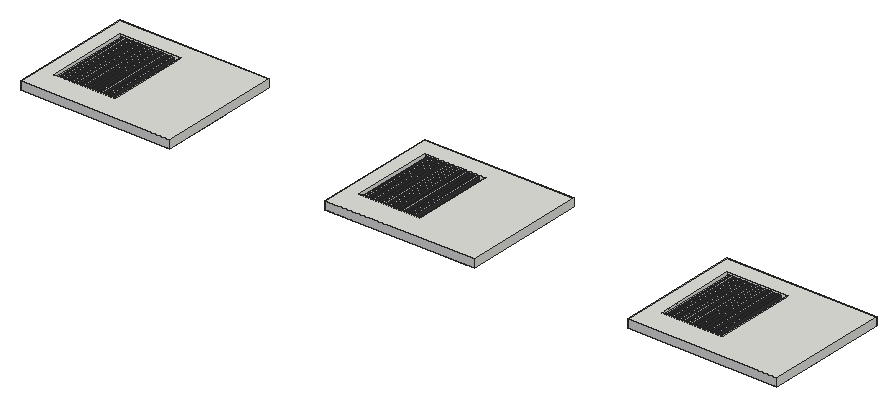
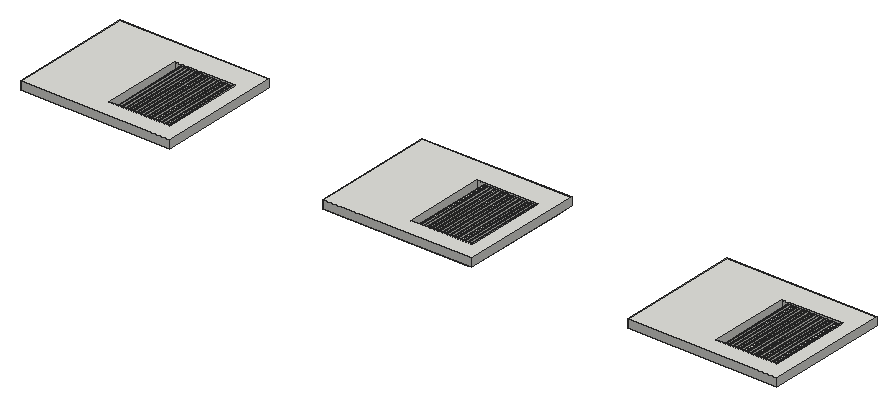
# SketchUp Ruby script. Lengths in inches.
U = 1.inch
M = Sketchup.active_model
def pt(a) = Geom::Point3d.new(a.map { |v| v * U })
def face(e, loops, mat)
  f = e.add_face(loops[0].map { |a| pt(a) })
  loops[1..].each { |l| e.add_face(l.map { |a| pt(a) }).erase! }
  f.material = f.back_material = mat if mat
  f
end
# faces: each face lists its corners as indices into pts; further lists are holes
def faces(e, pts, list, mat = nil) = list.each { |f| face(e, (f[0].is_a?(Array) ? f : [f]).map { |l| l.map { |i| pts[i] } }, mat) }
# xy, xz, yz: faces in a plane at the given z, y or x. An outline is a flat list of corners, or four numbers for a rectangle; further outlines are holes
def ring(l) = l.size == 4 ? [[l[0], l[1]], [l[2], l[1]], [l[2], l[3]], [l[0], l[3]]] : l.each_slice(2).to_a
def flat(e, list, mat, &to3) = list.each { |f| face(e, (f[0].is_a?(Array) ? f : [f]).map { |l| ring(l).map { |u, v| to3.(u, v) } }, mat) }
def xy(e, z, list, mat = nil) = flat(e, list, mat) { |x, y| [x, y, z] }
def xz(e, y, list, mat = nil) = flat(e, list, mat) { |x, z| [x, y, z] }
def yz(e, x, list, mat = nil) = flat(e, list, mat) { |y, z| [x, y, z] }
def lines(e, pts, list) = list.each { |a, b| e.add_line(pt(pts[a]), pt(pts[b])) }
# prism: a flat outline (further loops are holes) pulled along v
def prism(e, loops, v, mat = nil)
  f = face(e, loops, mat); d = Geom::Vector3d.new(v.map { |x| x * U })
  f.pushpull(f.normal.samedirection?(d) ? d.length : -d.length)
end
def box(e, o, s, mat = nil) = prism(e, [[o, [o[0] + s[0], o[1], o[2]], [o[0] + s[0], o[1] + s[1], o[2]], [o[0], o[1] + s[1], o[2]]]], [0, 0, s[2]], mat)
def at(x, y, z, deg = 0) = Geom::Transformation.translation(pt([x, y, z])) * Geom::Transformation.rotation(ORIGIN, Z_AXIS, deg.degrees)
def axes(o, x, y, z) = Geom::Transformation.new([*x, 0, *y, 0, *z, 0, *pt(o).to_a, 1])
def part(name) = M.definitions.add(name)
# library, detail: a bought-in or finely detailed component or shape, given as its bounding box
def library(name, o, s) = part(name).tap { |d| box(d.entities, o, s) }
def detail(e, o, s) = box(e.add_group.entities, o, s)
def put(e, d, t, mat = nil) = e.add_instance(d, t).tap { |i| i.material = mat if mat }
def group(e, t, mat = nil) = e.add_group.tap { |g| g.transformation = t; g.material = mat if mat }.entities
root = M.entities
M.materials.add("[Color M02]").color = [198, 198, 198]
M.materials.add("[Color M07]").color = [58, 58, 58]
xy(root,536.4375,[[1098.03,273.0625,1103.7,452.5625],[1103.7,273.0625,1103.7,308.24,1253.34,308.24,1253.34,273.0625,1249.29,273.0625,1249.29,289.5,1181.97,289.5,1181.97,273.0625],[1181.97,273.0625,1239.03,289.5],[1239.03,273.0625,1239.03,289.5,1249.29,273.0625],[1253.34,273.0625,1260.59,452.5625],
  [1884.4,273.0625,1890.08,452.5625],[1890.08,273.0625,1890.08,308.24,2039.72,308.24,2039.72,273.0625,2035.66,273.0625,2035.66,289.5,1968.34,289.5,1968.34,273.0625],[1968.34,273.0625,2025.4,289.5],[2025.4,273.0625,2025.4,289.5,2035.66,273.0625],[2039.72,273.0625,2046.96,452.5625],
  [2664.78,273.0625,2670.45,452.5625],[2670.45,273.0625,2670.45,308.24,2820.09,308.24,2820.09,273.0625,2816.04,273.0625,2816.04,289.5,2748.72,289.5,2748.72,273.0625],[2748.72,273.0625,2805.78,289.5],[2805.78,273.0625,2805.78,289.5,2816.04,273.0625],[2820.09,273.0625,2827.34,452.5625],
  [1103.7,308.24,1253.34,452.5625],[1890.08,308.24,2039.72,452.5625],[2670.45,308.24,2820.09,452.5625],[874.71,311.64,874.71,593.65,885.36,593.65,885.36,562.19,886.55,562.19,886.55,557.75,885.36,557.75,885.36,556.19,886.55,556.19,886.55,551.75,885.36,551.75,885.36,550.19,886.55,550.19,886.55,545.75,885.36,545.75,885.36,544.19,886.55,544.19,886.55,539.75,885.36,539.75,885.36,538.19,886.55,538.19,886.55,533.75,885.36,533.75,885.36,532.19,886.55,532.19,886.55,527.75,885.36,527.75,885.36,471.19,886.55,471.19,886.55,466.75,885.36,466.75,885.36,465.19,886.55,465.19,886.55,460.75,885.36,460.75,885.36,459.19,886.55,459.19,886.55,454.75,885.36,454.75,885.36,453.19,886.55,453.19,886.55,448.75,885.36,448.75,885.36,447.19,886.55,447.19,886.55,442.75,885.36,442.75,885.36,441.19,886.55,441.19,886.55,436.75,885.36,436.75,885.36,396.75,886.55,396.75,886.55,392.3125,885.36,392.3125,885.36,390.75,886.55,390.75,886.55,386.3125,885.36,386.3125,885.36,384.75,886.55,384.75,886.55,380.3125,885.36,380.3125,885.36,378.75,886.55,378.75,886.55,374.3125,885.36,374.3125,885.36,372.75,886.55,372.75,886.55,368.3125,885.36,368.3125,885.36,366.75,886.55,366.75,886.55,362.3125,885.36,362.3125,885.36,360.75,886.55,360.75,886.55,356.3125,885.36,356.3125,885.36,354.75,886.55,354.75,886.55,350.3125,885.36,350.3125,885.36,311.64],[1661.09,311.64,1661.09,593.65,1671.73,593.65,1671.73,562.19,1672.92,562.19,1672.92,557.75,1671.73,557.75,1671.73,556.19,1672.92,556.19,1672.92,551.75,1671.73,551.75,1671.73,550.19,1672.92,550.19,1672.92,545.75,1671.73,545.75,1671.73,544.19,1672.92,544.19,1672.92,539.75,1671.73,539.75,1671.73,538.19,1672.92,538.19,1672.92,533.75,1671.73,533.75,1671.73,532.19,1672.92,532.19,1672.92,527.75,1671.73,527.75,1671.73,471.19,1672.92,471.19,1672.92,466.75,1671.73,466.75,1671.73,465.19,1672.92,465.19,1672.92,460.75,1671.73,460.75,1671.73,459.19,1672.92,459.19,1672.92,454.75,1671.73,454.75,1671.73,453.19,1672.92,453.19,1672.92,448.75,1671.73,448.75,1671.73,447.19,1672.92,447.19,1672.92,442.75,1671.73,442.75,1671.73,441.19,1672.92,441.19,1672.92,436.75,1671.73,436.75,1671.73,396.75,1672.92,396.75,1672.92,392.3125,1671.73,392.3125,1671.73,390.75,1672.92,390.75,1672.92,386.3125,1671.73,386.3125,1671.73,384.75,1672.92,384.75,1672.92,380.3125,1671.73,380.3125,1671.73,378.75,1672.92,378.75,1672.92,374.3125,1671.73,374.3125,1671.73,372.75,1672.92,372.75,1672.92,368.3125,1671.73,368.3125,1671.73,366.75,1672.92,366.75,1672.92,362.3125,1671.73,362.3125,1671.73,360.75,1672.92,360.75,1672.92,356.3125,1671.73,356.3125,1671.73,354.75,1672.92,354.75,1672.92,350.3125,1671.73,350.3125,1671.73,311.64],
  [2441.46,311.64,2441.46,593.65,2452.11,593.65,2452.11,562.19,2453.3,562.19,2453.3,557.75,2452.11,557.75,2452.11,556.19,2453.3,556.19,2453.3,551.75,2452.11,551.75,2452.11,550.19,2453.3,550.19,2453.3,545.75,2452.11,545.75,2452.11,544.19,2453.3,544.19,2453.3,539.75,2452.11,539.75,2452.11,538.19,2453.3,538.19,2453.3,533.75,2452.11,533.75,2452.11,532.19,2453.3,532.19,2453.3,527.75,2452.11,527.75,2452.11,471.19,2453.3,471.19,2453.3,466.75,2452.11,466.75,2452.11,465.19,2453.3,465.19,2453.3,460.75,2452.11,460.75,2452.11,459.19,2453.3,459.19,2453.3,454.75,2452.11,454.75,2452.11,453.19,2453.3,453.19,2453.3,448.75,2452.11,448.75,2452.11,447.19,2453.3,447.19,2453.3,442.75,2452.11,442.75,2452.11,441.19,2453.3,441.19,2453.3,436.75,2452.11,436.75,2452.11,396.75,2453.3,396.75,2453.3,392.3125,2452.11,392.3125,2452.11,390.75,2453.3,390.75,2453.3,386.3125,2452.11,386.3125,2452.11,384.75,2453.3,384.75,2453.3,380.3125,2452.11,380.3125,2452.11,378.75,2453.3,378.75,2453.3,374.3125,2452.11,374.3125,2452.11,372.75,2453.3,372.75,2453.3,368.3125,2452.11,368.3125,2452.11,366.75,2453.3,366.75,2453.3,362.3125,2452.11,362.3125,2452.11,360.75,2453.3,360.75,2453.3,356.3125,2452.11,356.3125,2452.11,354.75,2453.3,354.75,2453.3,350.3125,2452.11,350.3125,2452.11,311.64],[1098.03,452.5625,1103.7,459.0625],[1103.7,452.5625,1260.59,459.0625],[1884.4,452.5625,1890.08,459.0625],[1890.08,452.5625,2046.96,459.0625],
  [2664.78,452.5625,2670.45,459.0625],[2670.45,452.5625,2827.34,459.0625]])
xy(root,536.4375,[[[874.71,273.0625,874.71,311.64,885.36,311.64,885.36,350.3125,886.55,350.3125,886.55,354.75,885.36,354.75,885.36,356.3125,886.55,356.3125,886.55,360.75,885.36,360.75,885.36,362.3125,886.55,362.3125,886.55,366.75,885.36,366.75,885.36,368.3125,886.55,368.3125,886.55,372.75,885.36,372.75,885.36,374.3125,886.55,374.3125,886.55,378.75,885.36,378.75,885.36,380.3125,886.55,380.3125,886.55,384.75,885.36,384.75,885.36,386.3125,886.55,386.3125,886.55,390.75,885.36,390.75,885.36,392.3125,886.55,392.3125,886.55,396.75,885.36,396.75,885.36,436.75,886.55,436.75,886.55,441.19,885.36,441.19,885.36,442.75,886.55,442.75,886.55,447.19,885.36,447.19,885.36,448.75,886.55,448.75,886.55,453.19,885.36,453.19,885.36,454.75,886.55,454.75,886.55,459.19,885.36,459.19,885.36,460.75,886.55,460.75,886.55,465.19,885.36,465.19,885.36,466.75,886.55,466.75,886.55,471.19,885.36,471.19,885.36,527.75,886.55,527.75,886.55,532.19,885.36,532.19,885.36,533.75,886.55,533.75,886.55,538.19,885.36,538.19,885.36,539.75,886.55,539.75,886.55,544.19,885.36,544.19,885.36,545.75,886.55,545.75,886.55,550.19,885.36,550.19,885.36,551.75,886.55,551.75,886.55,556.19,885.36,556.19,885.36,557.75,886.55,557.75,886.55,562.19,885.36,562.19,885.36,593.65,1260.59,593.65,1260.59,459.0625,1098.03,459.0625,1098.03,273.0625],[911.37,336.64,1067.68,548.95]],[[1661.09,273.0625,1661.09,311.64,1671.73,311.64,1671.73,350.3125,1672.92,350.3125,1672.92,354.75,1671.73,354.75,1671.73,356.3125,1672.92,356.3125,1672.92,360.75,1671.73,360.75,1671.73,362.3125,1672.92,362.3125,1672.92,366.75,1671.73,366.75,1671.73,368.3125,1672.92,368.3125,1672.92,372.75,1671.73,372.75,1671.73,374.3125,1672.92,374.3125,1672.92,378.75,1671.73,378.75,1671.73,380.3125,1672.92,380.3125,1672.92,384.75,1671.73,384.75,1671.73,386.3125,1672.92,386.3125,1672.92,390.75,1671.73,390.75,1671.73,392.3125,1672.92,392.3125,1672.92,396.75,1671.73,396.75,1671.73,436.75,1672.92,436.75,1672.92,441.19,1671.73,441.19,1671.73,442.75,1672.92,442.75,1672.92,447.19,1671.73,447.19,1671.73,448.75,1672.92,448.75,1672.92,453.19,1671.73,453.19,1671.73,454.75,1672.92,454.75,1672.92,459.19,1671.73,459.19,1671.73,460.75,1672.92,460.75,1672.92,465.19,1671.73,465.19,1671.73,466.75,1672.92,466.75,1672.92,471.19,1671.73,471.19,1671.73,527.75,1672.92,527.75,1672.92,532.19,1671.73,532.19,1671.73,533.75,1672.92,533.75,1672.92,538.19,1671.73,538.19,1671.73,539.75,1672.92,539.75,1672.92,544.19,1671.73,544.19,1671.73,545.75,1672.92,545.75,1672.92,550.19,1671.73,550.19,1671.73,551.75,1672.92,551.75,1672.92,556.19,1671.73,556.19,1671.73,557.75,1672.92,557.75,1672.92,562.19,1671.73,562.19,1671.73,593.65,2046.96,593.65,2046.96,459.0625,1884.4,459.0625,1884.4,273.0625],[1697.74,336.64,1854.06,548.95]],[[2441.46,273.0625,2441.46,311.64,2452.11,311.64,2452.11,350.3125,2453.3,350.3125,2453.3,354.75,2452.11,354.75,2452.11,356.3125,2453.3,356.3125,2453.3,360.75,2452.11,360.75,2452.11,362.3125,2453.3,362.3125,2453.3,366.75,2452.11,366.75,2452.11,368.3125,2453.3,368.3125,2453.3,372.75,2452.11,372.75,2452.11,374.3125,2453.3,374.3125,2453.3,378.75,2452.11,378.75,2452.11,380.3125,2453.3,380.3125,2453.3,384.75,2452.11,384.75,2452.11,386.3125,2453.3,386.3125,2453.3,390.75,2452.11,390.75,2452.11,392.3125,2453.3,392.3125,2453.3,396.75,2452.11,396.75,2452.11,436.75,2453.3,436.75,2453.3,441.19,2452.11,441.19,2452.11,442.75,2453.3,442.75,2453.3,447.19,2452.11,447.19,2452.11,448.75,2453.3,448.75,2453.3,453.19,2452.11,453.19,2452.11,454.75,2453.3,454.75,2453.3,459.19,2452.11,459.19,2452.11,460.75,2453.3,460.75,2453.3,465.19,2452.11,465.19,2452.11,466.75,2453.3,466.75,2453.3,471.19,2452.11,471.19,2452.11,527.75,2453.3,527.75,2453.3,532.19,2452.11,532.19,2452.11,533.75,2453.3,533.75,2453.3,538.19,2452.11,538.19,2452.11,539.75,2453.3,539.75,2453.3,544.19,2452.11,544.19,2452.11,545.75,2453.3,545.75,2453.3,550.19,2452.11,550.19,2452.11,551.75,2453.3,551.75,2453.3,556.19,2452.11,556.19,2452.11,557.75,2453.3,557.75,2453.3,562.19,2452.11,562.19,2452.11,593.65,2827.34,593.65,2827.34,459.0625,2664.78,459.0625,2664.78,273.0625],[2478.12,336.64,2634.43,548.95]]],"[Color M02]")
xy(root,540.1,[[915.63,336.64,920.38,548.95],[924.38,336.64,929.13,548.95],[933.76,336.64,938.51,548.95],[943.13,336.64,947.88,548.95],[952.51,336.64,957.26,548.95],
  [961.88,336.64,966.63,548.95],[971.26,336.64,976.01,548.95],[980.63,336.64,985.38,548.95],[990.01,336.64,994.76,548.95],[999.38,336.64,1004.13,548.95],
  [1008.76,336.64,1013.51,548.95],[1018.13,336.64,1022.88,548.95],[1027.51,336.64,1032.26,548.95],[1036.88,336.64,1041.63,548.95],[1046.26,336.64,1051.01,548.95],
  [1702.01,336.64,1706.76,548.95],[1710.76,336.64,1715.51,548.95],[1720.13,336.64,1724.88,548.95],[1729.51,336.64,1734.26,548.95],[1738.88,336.64,1743.63,548.95],
  [1748.26,336.64,1753.01,548.95],[1757.63,336.64,1762.38,548.95],[1767.01,336.64,1771.76,548.95],[1776.38,336.64,1781.13,548.95],[1785.76,336.64,1790.51,548.95],
  [1795.13,336.64,1799.88,548.95],[1804.51,336.64,1809.26,548.95],[1813.88,336.64,1818.63,548.95],[1823.26,336.64,1828.01,548.95],[1832.63,336.64,1837.38,548.95],
  [2482.38,336.64,2487.13,548.95],[2491.13,336.64,2495.88,548.95],[2500.51,336.64,2505.26,548.95],[2509.88,336.64,2514.63,548.95],[2519.26,336.64,2524.01,548.95],
  [2528.63,336.64,2533.38,548.95],[2538.01,336.64,2542.76,548.95],[2547.38,336.64,2552.13,548.95],[2556.76,336.64,2561.51,548.95],[2566.13,336.64,2570.88,548.95],
  [2575.51,336.64,2580.26,548.95],[2584.88,336.64,2589.63,548.95],[2594.26,336.64,2599.01,548.95],[2603.63,336.64,2608.38,548.95],[2613.01,336.64,2617.76,548.95]],"[Color M07]")
xy(root,552.16,[[915.63,336.64,920.38,548.95],[924.38,336.64,929.13,548.95],[933.76,336.64,938.51,548.95],[943.13,336.64,947.88,548.95],[952.51,336.64,957.26,548.95],
  [961.88,336.64,966.63,548.95],[971.26,336.64,976.01,548.95],[980.63,336.64,985.38,548.95],[990.01,336.64,994.76,548.95],[999.38,336.64,1004.13,548.95],
  [1008.76,336.64,1013.51,548.95],[1018.13,336.64,1022.88,548.95],[1027.51,336.64,1032.26,548.95],[1036.88,336.64,1041.63,548.95],[1046.26,336.64,1051.01,548.95],
  [1702.01,336.64,1706.76,548.95],[1710.76,336.64,1715.51,548.95],[1720.13,336.64,1724.88,548.95],[1729.51,336.64,1734.26,548.95],[1738.88,336.64,1743.63,548.95],
  [1748.26,336.64,1753.01,548.95],[1757.63,336.64,1762.38,548.95],[1767.01,336.64,1771.76,548.95],[1776.38,336.64,1781.13,548.95],[1785.76,336.64,1790.51,548.95],
  [1795.13,336.64,1799.88,548.95],[1804.51,336.64,1809.26,548.95],[1813.88,336.64,1818.63,548.95],[1823.26,336.64,1828.01,548.95],[1832.63,336.64,1837.38,548.95],
  [2482.38,336.64,2487.13,548.95],[2491.13,336.64,2495.88,548.95],[2500.51,336.64,2505.26,548.95],[2509.88,336.64,2514.63,548.95],[2519.26,336.64,2524.01,548.95],
  [2528.63,336.64,2533.38,548.95],[2538.01,336.64,2542.76,548.95],[2547.38,336.64,2552.13,548.95],[2556.76,336.64,2561.51,548.95],[2566.13,336.64,2570.88,548.95],
  [2575.51,336.64,2580.26,548.95],[2584.88,336.64,2589.63,548.95],[2594.26,336.64,2599.01,548.95],[2603.63,336.64,2608.38,548.95],[2613.01,336.64,2617.76,548.95]])
xy(root,557.1875,[[[874.71,273.0625,1260.59,593.65],[911.37,336.64,1067.68,548.95]],[[1661.09,273.0625,2046.96,593.65],[1697.74,336.64,1854.06,548.95]],[[2441.46,273.0625,2827.34,593.65],[2478.12,336.64,2634.43,548.95]]])
xz(root,273.0625,[[874.71,536.4375,1260.59,557.1875],[1661.09,536.4375,2046.96,557.1875],[2441.46,536.4375,2827.34,557.1875]],"[Color M02]")
xz(root,336.64,[[[911.37,536.4375,1067.68,557.1875],[1018.13,540.1,1022.88,552.16],[915.63,540.1,920.38,552.16],[924.38,540.1,929.13,552.16],[933.76,540.1,938.51,552.16],[943.13,540.1,947.88,552.16],[952.51,540.1,957.26,552.16],[961.88,540.1,966.63,552.16],[971.26,540.1,976.01,552.16],[980.63,540.1,985.38,552.16],[990.01,540.1,994.76,552.16],[999.38,540.1,1004.13,552.16],[1008.76,540.1,1013.51,552.16],[1027.51,540.1,1032.26,552.16],[1036.88,540.1,1041.63,552.16],[1046.26,540.1,1051.01,552.16]],[[1697.74,536.4375,1854.06,557.1875],[1804.51,540.1,1809.26,552.16],[1702.01,540.1,1706.76,552.16],[1710.76,540.1,1715.51,552.16],[1720.13,540.1,1724.88,552.16],[1729.51,540.1,1734.26,552.16],[1738.88,540.1,1743.63,552.16],[1748.26,540.1,1753.01,552.16],[1757.63,540.1,1762.38,552.16],[1767.01,540.1,1771.76,552.16],[1776.38,540.1,1781.13,552.16],[1785.76,540.1,1790.51,552.16],[1795.13,540.1,1799.88,552.16],[1813.88,540.1,1818.63,552.16],[1823.26,540.1,1828.01,552.16],[1832.63,540.1,1837.38,552.16]],[[2478.12,536.4375,2634.43,557.1875],[2482.38,540.1,2487.13,552.16],[2491.13,540.1,2495.88,552.16],[2500.51,540.1,2505.26,552.16],[2509.88,540.1,2514.63,552.16],[2519.26,540.1,2524.01,552.16],[2528.63,540.1,2533.38,552.16],[2538.01,540.1,2542.76,552.16],[2547.38,540.1,2552.13,552.16],[2556.76,540.1,2561.51,552.16],[2566.13,540.1,2570.88,552.16],[2575.51,540.1,2580.26,552.16],[2584.88,540.1,2589.63,552.16],[2594.26,540.1,2599.01,552.16],[2603.63,540.1,2608.38,552.16],[2613.01,540.1,2617.76,552.16]]])
xz(root,548.95,[[[911.37,536.4375,1067.68,557.1875],[1018.13,540.1,1022.88,552.16],[915.63,540.1,920.38,552.16],[924.38,540.1,929.13,552.16],[933.76,540.1,938.51,552.16],[943.13,540.1,947.88,552.16],[952.51,540.1,957.26,552.16],[961.88,540.1,966.63,552.16],[971.26,540.1,976.01,552.16],[980.63,540.1,985.38,552.16],[990.01,540.1,994.76,552.16],[999.38,540.1,1004.13,552.16],[1008.76,540.1,1013.51,552.16],[1027.51,540.1,1032.26,552.16],[1036.88,540.1,1041.63,552.16],[1046.26,540.1,1051.01,552.16]],[[1697.74,536.4375,1854.06,557.1875],[1804.51,540.1,1809.26,552.16],[1702.01,540.1,1706.76,552.16],[1710.76,540.1,1715.51,552.16],[1720.13,540.1,1724.88,552.16],[1729.51,540.1,1734.26,552.16],[1738.88,540.1,1743.63,552.16],[1748.26,540.1,1753.01,552.16],[1757.63,540.1,1762.38,552.16],[1767.01,540.1,1771.76,552.16],[1776.38,540.1,1781.13,552.16],[1785.76,540.1,1790.51,552.16],[1795.13,540.1,1799.88,552.16],[1813.88,540.1,1818.63,552.16],[1823.26,540.1,1828.01,552.16],[1832.63,540.1,1837.38,552.16]],[[2478.12,536.4375,2634.43,557.1875],[2482.38,540.1,2487.13,552.16],[2491.13,540.1,2495.88,552.16],[2500.51,540.1,2505.26,552.16],[2509.88,540.1,2514.63,552.16],[2519.26,540.1,2524.01,552.16],[2528.63,540.1,2533.38,552.16],[2538.01,540.1,2542.76,552.16],[2547.38,540.1,2552.13,552.16],[2556.76,540.1,2561.51,552.16],[2566.13,540.1,2570.88,552.16],[2575.51,540.1,2580.26,552.16],[2584.88,540.1,2589.63,552.16],[2594.26,540.1,2599.01,552.16],[2603.63,540.1,2608.38,552.16],[2613.01,540.1,2617.76,552.16]]])
xz(root,593.65,[[874.71,536.4375,1260.59,557.1875],[1661.09,536.4375,2046.96,557.1875],[2441.46,536.4375,2827.34,557.1875]])
yz(root,874.71,[[273.0625,536.4375,593.65,557.1875]])
yz(root,911.37,[[336.64,536.4375,548.95,557.1875]])
yz(root,915.63,[[336.64,540.1,548.95,552.16]])
yz(root,920.38,[[336.64,540.1,548.95,552.16]],"[Color M07]")
yz(root,924.38,[[336.64,540.1,548.95,552.16]])
yz(root,929.13,[[336.64,540.1,548.95,552.16]],"[Color M07]")
yz(root,933.76,[[336.64,540.1,548.95,552.16]])
yz(root,938.51,[[336.64,540.1,548.95,552.16]],"[Color M07]")
yz(root,943.13,[[336.64,540.1,548.95,552.16]])
yz(root,947.88,[[336.64,540.1,548.95,552.16]],"[Color M07]")
yz(root,952.51,[[336.64,540.1,548.95,552.16]])
yz(root,957.26,[[336.64,540.1,548.95,552.16]],"[Color M07]")
yz(root,961.88,[[336.64,540.1,548.95,552.16]])
yz(root,966.63,[[336.64,540.1,548.95,552.16]],"[Color M07]")
yz(root,971.26,[[336.64,540.1,548.95,552.16]])
yz(root,976.01,[[336.64,540.1,548.95,552.16]],"[Color M07]")
yz(root,980.63,[[336.64,540.1,548.95,552.16]])
yz(root,985.38,[[336.64,540.1,548.95,552.16]],"[Color M07]")
yz(root,990.01,[[336.64,540.1,548.95,552.16]])
yz(root,994.76,[[336.64,540.1,548.95,552.16]],"[Color M07]")
yz(root,999.38,[[336.64,540.1,548.95,552.16]])
yz(root,1004.13,[[336.64,540.1,548.95,552.16]],"[Color M07]")
yz(root,1008.76,[[336.64,540.1,548.95,552.16]])
yz(root,1013.51,[[336.64,540.1,548.95,552.16]],"[Color M07]")
yz(root,1018.13,[[336.64,540.1,548.95,552.16]])
yz(root,1022.88,[[336.64,540.1,548.95,552.16]],"[Color M07]")
yz(root,1027.51,[[336.64,540.1,548.95,552.16]])
yz(root,1032.26,[[336.64,540.1,548.95,552.16]],"[Color M07]")
yz(root,1036.88,[[336.64,540.1,548.95,552.16]])
yz(root,1041.63,[[336.64,540.1,548.95,552.16]],"[Color M07]")
yz(root,1046.26,[[336.64,540.1,548.95,552.16]])
yz(root,1051.01,[[336.64,540.1,548.95,552.16]],"[Color M07]")
yz(root,1067.68,[[336.64,536.4375,548.95,557.1875]])
yz(root,1260.59,[[273.0625,536.4375,593.65,557.1875]])
yz(root,1661.09,[[273.0625,536.4375,593.65,557.1875]])
yz(root,1697.74,[[336.64,536.4375,548.95,557.1875]])
yz(root,1702.01,[[336.64,540.1,548.95,552.16]])
yz(root,1706.76,[[336.64,540.1,548.95,552.16]],"[Color M07]")
yz(root,1710.76,[[336.64,540.1,548.95,552.16]])
yz(root,1715.51,[[336.64,540.1,548.95,552.16]],"[Color M07]")
yz(root,1720.13,[[336.64,540.1,548.95,552.16]])
yz(root,1724.88,[[336.64,540.1,548.95,552.16]],"[Color M07]")
yz(root,1729.51,[[336.64,540.1,548.95,552.16]])
yz(root,1734.26,[[336.64,540.1,548.95,552.16]],"[Color M07]")
yz(root,1738.88,[[336.64,540.1,548.95,552.16]])
yz(root,1743.63,[[336.64,540.1,548.95,552.16]],"[Color M07]")
yz(root,1748.26,[[336.64,540.1,548.95,552.16]])
yz(root,1753.01,[[336.64,540.1,548.95,552.16]],"[Color M07]")
yz(root,1757.63,[[336.64,540.1,548.95,552.16]])
yz(root,1762.38,[[336.64,540.1,548.95,552.16]],"[Color M07]")
yz(root,1767.01,[[336.64,540.1,548.95,552.16]])
yz(root,1771.76,[[336.64,540.1,548.95,552.16]],"[Color M07]")
yz(root,1776.38,[[336.64,540.1,548.95,552.16]])
yz(root,1781.13,[[336.64,540.1,548.95,552.16]],"[Color M07]")
yz(root,1785.76,[[336.64,540.1,548.95,552.16]])
yz(root,1790.51,[[336.64,540.1,548.95,552.16]],"[Color M07]")
yz(root,1795.13,[[336.64,540.1,548.95,552.16]])
yz(root,1799.88,[[336.64,540.1,548.95,552.16]],"[Color M07]")
yz(root,1804.51,[[336.64,540.1,548.95,552.16]])
yz(root,1809.26,[[336.64,540.1,548.95,552.16]],"[Color M07]")
yz(root,1813.88,[[336.64,540.1,548.95,552.16]])
yz(root,1818.63,[[336.64,540.1,548.95,552.16]],"[Color M07]")
yz(root,1823.26,[[336.64,540.1,548.95,552.16]])
yz(root,1828.01,[[336.64,540.1,548.95,552.16]],"[Color M07]")
yz(root,1832.63,[[336.64,540.1,548.95,552.16]])
yz(root,1837.38,[[336.64,540.1,548.95,552.16]],"[Color M07]")
yz(root,1854.06,[[336.64,536.4375,548.95,557.1875]])
yz(root,2046.96,[[273.0625,536.4375,593.65,557.1875]])
yz(root,2441.46,[[273.0625,536.4375,593.65,557.1875]])
yz(root,2478.12,[[336.64,536.4375,548.95,557.1875]])
yz(root,2482.38,[[336.64,540.1,548.95,552.16]])
yz(root,2487.13,[[336.64,540.1,548.95,552.16]],"[Color M07]")
yz(root,2491.13,[[336.64,540.1,548.95,552.16]])
yz(root,2495.88,[[336.64,540.1,548.95,552.16]],"[Color M07]")
yz(root,2500.51,[[336.64,540.1,548.95,552.16]])
yz(root,2505.26,[[336.64,540.1,548.95,552.16]],"[Color M07]")
yz(root,2509.88,[[336.64,540.1,548.95,552.16]])
yz(root,2514.63,[[336.64,540.1,548.95,552.16]],"[Color M07]")
yz(root,2519.26,[[336.64,540.1,548.95,552.16]])
yz(root,2524.01,[[336.64,540.1,548.95,552.16]],"[Color M07]")
yz(root,2528.63,[[336.64,540.1,548.95,552.16]])
yz(root,2533.38,[[336.64,540.1,548.95,552.16]],"[Color M07]")
yz(root,2538.01,[[336.64,540.1,548.95,552.16]])
yz(root,2542.76,[[336.64,540.1,548.95,552.16]],"[Color M07]")
yz(root,2547.38,[[336.64,540.1,548.95,552.16]])
yz(root,2552.13,[[336.64,540.1,548.95,552.16]],"[Color M07]")
yz(root,2556.76,[[336.64,540.1,548.95,552.16]])
yz(root,2561.51,[[336.64,540.1,548.95,552.16]],"[Color M07]")
yz(root,2566.13,[[336.64,540.1,548.95,552.16]])
yz(root,2570.88,[[336.64,540.1,548.95,552.16]],"[Color M07]")
yz(root,2575.51,[[336.64,540.1,548.95,552.16]])
yz(root,2580.26,[[336.64,540.1,548.95,552.16]],"[Color M07]")
yz(root,2584.88,[[336.64,540.1,548.95,552.16]])
yz(root,2589.63,[[336.64,540.1,548.95,552.16]],"[Color M07]")
yz(root,2594.26,[[336.64,540.1,548.95,552.16]])
yz(root,2599.01,[[336.64,540.1,548.95,552.16]],"[Color M07]")
yz(root,2603.63,[[336.64,540.1,548.95,552.16]])
yz(root,2608.38,[[336.64,540.1,548.95,552.16]],"[Color M07]")
yz(root,2613.01,[[336.64,540.1,548.95,552.16]])
yz(root,2617.76,[[336.64,540.1,548.95,552.16]],"[Color M07]")
yz(root,2634.43,[[336.64,536.4375,548.95,557.1875]])
yz(root,2827.34,[[273.0625,536.4375,593.65,557.1875]])
p = [[1671.73,301,536.4375],[1671.73,311.64,536.4375],[885.36,301,536.4375],[885.36,311.64,536.4375],[2452.11,301,536.4375],[2452.11,311.64,536.4375]]
lines(root,p,[[0,1],[2,3],[4,5]])
